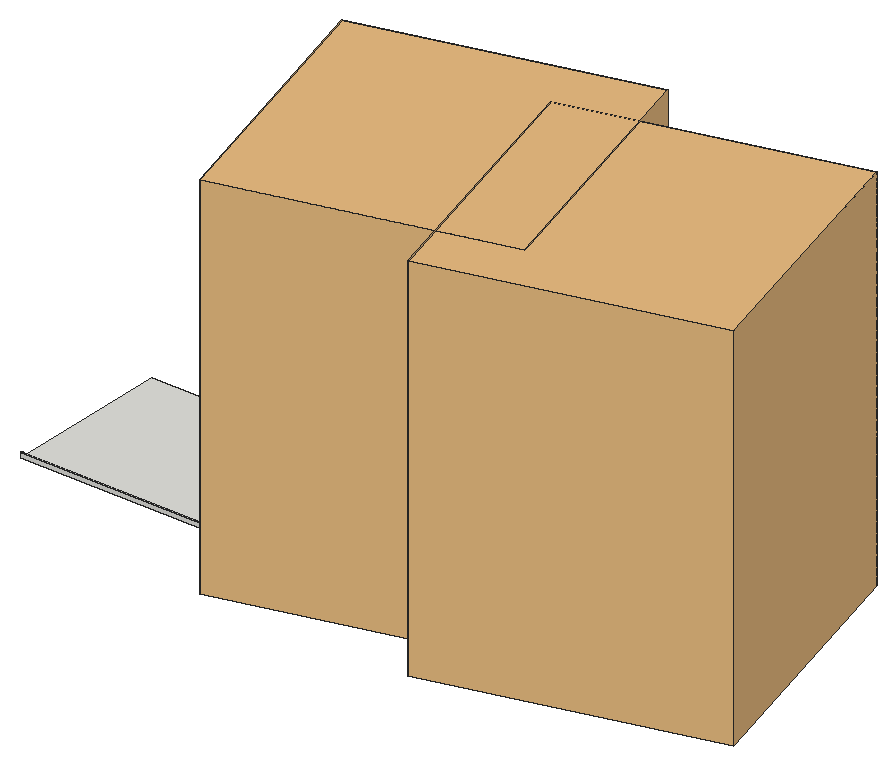
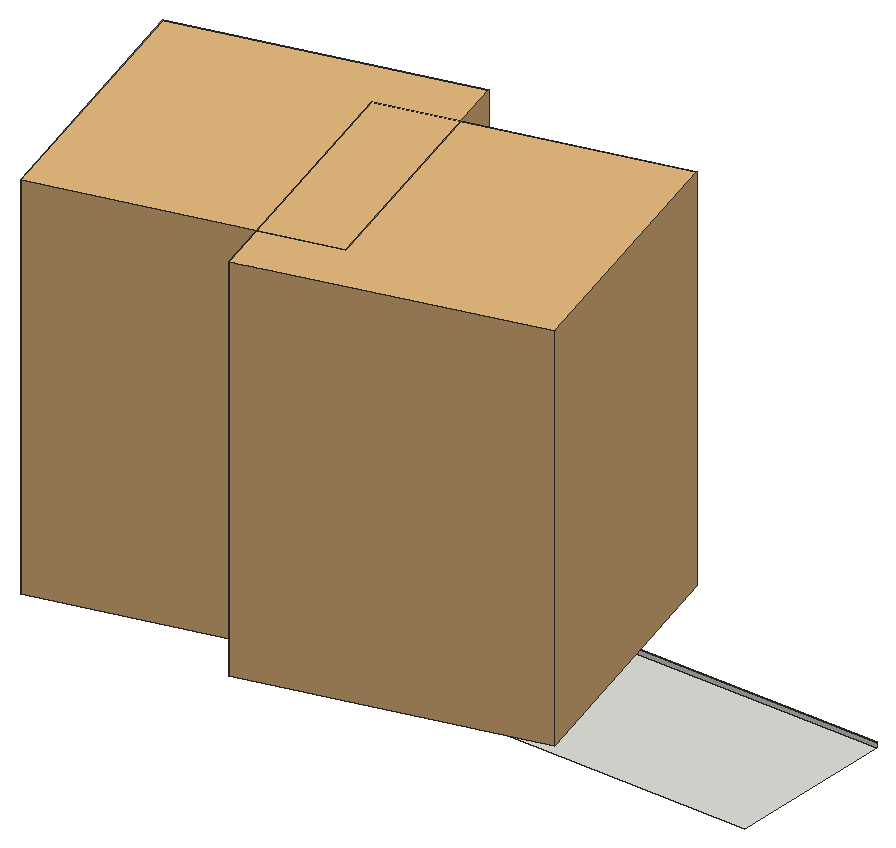
# SketchUp Ruby script. Lengths in inches.
U = 1.inch
M = Sketchup.active_model
def pt(a) = Geom::Point3d.new(a.map { |v| v * U })
def face(e, loops, mat)
  f = e.add_face(loops[0].map { |a| pt(a) })
  loops[1..].each { |l| e.add_face(l.map { |a| pt(a) }).erase! }
  f.material = f.back_material = mat if mat
  f
end
# faces: each face lists its corners as indices into pts; further lists are holes
def faces(e, pts, list, mat = nil) = list.each { |f| face(e, (f[0].is_a?(Array) ? f : [f]).map { |l| l.map { |i| pts[i] } }, mat) }
# xy, xz, yz: faces in a plane at the given z, y or x. An outline is a flat list of corners, or four numbers for a rectangle; further outlines are holes
def ring(l) = l.size == 4 ? [[l[0], l[1]], [l[2], l[1]], [l[2], l[3]], [l[0], l[3]]] : l.each_slice(2).to_a
def flat(e, list, mat, &to3) = list.each { |f| face(e, (f[0].is_a?(Array) ? f : [f]).map { |l| ring(l).map { |u, v| to3.(u, v) } }, mat) }
def xy(e, z, list, mat = nil) = flat(e, list, mat) { |x, y| [x, y, z] }
def xz(e, y, list, mat = nil) = flat(e, list, mat) { |x, z| [x, y, z] }
def yz(e, x, list, mat = nil) = flat(e, list, mat) { |y, z| [x, y, z] }
def lines(e, pts, list) = list.each { |a, b| e.add_line(pt(pts[a]), pt(pts[b])) }
# prism: a flat outline (further loops are holes) pulled along v
def prism(e, loops, v, mat = nil)
  f = face(e, loops, mat); d = Geom::Vector3d.new(v.map { |x| x * U })
  f.pushpull(f.normal.samedirection?(d) ? d.length : -d.length)
end
def box(e, o, s, mat = nil) = prism(e, [[o, [o[0] + s[0], o[1], o[2]], [o[0] + s[0], o[1] + s[1], o[2]], [o[0], o[1] + s[1], o[2]]]], [0, 0, s[2]], mat)
def at(x, y, z, deg = 0) = Geom::Transformation.translation(pt([x, y, z])) * Geom::Transformation.rotation(ORIGIN, Z_AXIS, deg.degrees)
def axes(o, x, y, z) = Geom::Transformation.new([*x, 0, *y, 0, *z, 0, *pt(o).to_a, 1])
def part(name) = M.definitions.add(name)
# library, detail: a bought-in or finely detailed component or shape, given as its bounding box
def library(name, o, s) = part(name).tap { |d| box(d.entities, o, s) }
def detail(e, o, s) = box(e.add_group.entities, o, s)
def put(e, d, t, mat = nil) = e.add_instance(d, t).tap { |i| i.material = mat if mat }
def group(e, t, mat = nil) = e.add_group.tap { |g| g.transformation = t; g.material = mat if mat }.entities
root = M.entities
M.materials.add("Material82").color = [68, 110, 58]
M.materials.add("Material83").color = [48, 90, 38]
M.materials.add("Material84").color = [68, 110, 48]
M.materials.add("Material85").color = [48, 90, 48]
M.materials.add("Material86").color = [58, 110, 58]
M.materials.add("Material87").color = [58, 90, 38]
M.materials.add("Material88").color = [68, 100, 58]
M.materials.add("Material89").color = [48, 100, 38]
c1 = part("grass00")
p = [[-0.6875,0.15,0],[-0.56,0.08,5.52],[-0.04,0.03,2.76],[0.48,-0.02,0],[0.35,-0.02,5.52],[-0.1,-0.14,5.52],
  [-0.12,0.65,8.37],[-0.42,0.65,8.37]]
faces(c1.entities,p,[[0,1,2,3],[3,2,4],[1,5,2],[5,4,2],[1,6,5],[4,5,6],[7,6,1]])
c2 = part("Group16\#1")
put(c2.entities,c1,axes([1.44,-0.61,-0.01],[0.05352,0.12609,0],[-0.10704,0.04543,0.07239],[0.06664,-0.02828,0.11628]),"Material85")
put(c2.entities,c1,axes([0.76,-0.15,-0.01],[0.04676,0.24062,0],[-0.23162,0.04501,0.06642],[0.0652,-0.01267,0.23595]),"Material82")
put(c2.entities,c1,axes([0.79,0.01,-0.01],[-0.00606,0.34651,0],[-0.34381,-0.00602,0.0432],[0.04319,0.00076,0.34386]))
put(c2.entities,c1,axes([1,0.23,-0.01],[-0.07192,0.31144,0],[-0.28722,-0.06632,0.1236],[0.12043,0.02781,0.29478]),"Material84")
put(c2.entities,c1,axes([1.66,0.77,-0.01],[-0.13828,0.29651,0],[-0.21551,-0.1005,0.22471],[0.20365,0.09498,0.23779]),"Material89")
put(c2.entities,c1,axes([0.6875,0.52,-0.01],[-0.18126,0.24051,0],[-0.22746,-0.17142,0.09788],[0.07817,0.05891,0.28481]),"Material84")
put(c2.entities,c1,axes([0.68,0.78,-0.01],[-0.215,0.18688,0],[-0.12385,-0.14248,0.21334],[0.13995,0.16101,0.18878]),"Material82")
put(c2.entities,c1,axes([0.56,1,-0.01],[-0.13756,0.07624,0],[-0.06159,-0.11112,0.0927],[0.04494,0.08108,0.12705]),"Material84")
put(c2.entities,c1,axes([0.2,0.64,-0.01],[-0.23729,0.07254,0],[-0.05711,-0.18681,0.153],[0.04473,0.14632,0.19535]),"Material89")
put(c2.entities,c1,axes([0.0625,0.72,-0.01],[-0.28874,0.02525,0],[-0.02179,-0.24916,0.14647],[0.01276,0.14591,0.25012]),"Material82")
put(c2.entities,c1,axes([-0.08,0.62,-0.01],[-0.34089,-0.04187,0],[0.03255,-0.26504,0.216],[-0.02633,0.21439,0.26703]),"Material89")
put(c2.entities,c1,axes([-0.34,0.98,-0.01],[-0.14314,-0.0493,0],[0.04397,-0.12769,0.06843],[-0.02228,0.0647,0.13505]),"Material89")
put(c2.entities,c1,axes([-0.87,1.45,-0.01],[-0.23488,-0.14114,0],[0.13761,-0.22901,0.06087],[-0.03135,0.05217,0.26717]))
put(c2.entities,c1,axes([-0.72,0.77,-0.01],[-0.14208,-0.13251,0],[0.07209,-0.0773,0.16301],[-0.11118,0.11922,0.1057]),"Material89")
put(c2.entities,c1,axes([-0.62,0.43,-0.01],[-0.14845,-0.21203,0],[0.18654,-0.13061,0.12304],[-0.10079,0.07057,0.22772]),"Material82")
put(c2.entities,c1,axes([-0.68,0.29,-0.01],[-0.13639,-0.32136,0],[0.31723,-0.13464,0.05579],[-0.05136,0.0218,0.34462]),"Material83")
put(c2.entities,c1,axes([-0.64,0.125,-0.01],[-0.0458,-0.23569,0],[0.22124,-0.043,0.08276],[-0.08124,0.01579,0.22538]),"Material86")
put(c2.entities,c1,axes([-1.6,-0.03,-0.01],[0.00576,-0.32897,0],[0.27526,0.00482,0.18018],[-0.18015,-0.00315,0.2753]),"Material84")
put(c2.entities,c1,axes([-1.36,-0.31,-0.01],[0.05718,-0.24765,0],[0.18172,0.04196,0.17267],[-0.16825,-0.03885,0.1865]),"Material89")
put(c2.entities,c1,axes([-1.54,-0.72,-0.01],[0.06537,-0.14017,0],[0.13555,0.06321,0.03939],[-0.0357,-0.01665,0.14956]))
put(c2.entities,c1,axes([-1.19,-0.9,-0.01],[0.09597,-0.12735,0],[0.11214,0.08451,0.07557],[-0.06035,-0.04548,0.14042]),"Material88")
put(c2.entities,c1,axes([-0.47,-0.54,-0.01],[0.11588,-0.10072,0],[0.0618,0.0711,0.12124],[-0.07953,-0.0915,0.0942]))
put(c2.entities,c1,axes([-0.47,-0.84,-0.01],[0.11927,-0.0661,0],[0.06603,0.11913,0.00646],[-0.00313,-0.00565,0.13621]),"Material84")
put(c2.entities,c1,axes([-0.38,-1.24,-0.01],[0.28037,-0.08571,0],[0.0618,0.20215,0.20315],[-0.05939,-0.19428,0.21139]),"Material88")
put(c2.entities,c1,axes([-0.06,-0.66,-0.01],[0.22719,-0.01987,0],[0.01247,0.14255,0.17758],[-0.01547,-0.17691,0.1431]),"Material87")
put(c2.entities,c1,axes([0.11,-0.89,-0.01],[0.14882,0.01828,0],[-0.01058,0.08611,0.12229],[0.01491,-0.12138,0.08676]),"Material85")
put(c2.entities,c1,axes([0.25,-0.72,-0.01],[0.20481,0.07053,0],[-0.06206,0.18022,0.10291],[0.03351,-0.0973,0.1906]),"Material85")
put(c2.entities,c1,axes([0.85,-1.42,-0.01],[0.16481,0.09904,0],[-0.09472,0.15762,0.05616],[0.02893,-0.04814,0.18389]),"Material84")
put(c2.entities,c1,axes([1.01,-1.09,-0.01],[0.21858,0.20385,0],[-0.17495,0.1876,0.15339],[0.10462,-0.11218,0.25652]),"Material89")
put(c2.entities,c1,axes([1.01,-0.71,-0.01],[0.08733,0.12473,0],[-0.06445,0.04512,0.13037],[0.1068,-0.07477,0.07867]),"Material85")
c3 = part("Group15\#1")
put(c3.entities,c2,at(0,0,0))
c4 = part("3darcstudiotree_grass00\#1")
put(c4.entities,c3,at(0,0,0))
c5 = library("Palm tree",[-4.09,-4.52,0],[193.52,193.51,258.93])
c6 = part("Palm+Tree")
put(c6.entities,c5,at(25.51,-21.81,0,15))
c7 = library("Group\#612",[0,0,0],[32.91,53.52,103.45])
xy(root,-42.1875,[[626.68,273.41,1048.66,387.84]])
xz(root,273.41,[[626.68,-42.1875,1048.66,-42.1875,1048.66,-38.61,848.97,-38.61,848.97,-39.125,626.68,-39.125],[626.68,-38.61,1048.66,-38.1875]])
put(root,c4,axes([808.61,334.13,-34.17],[-3.94658,0.83198,0],[-2.08533,-1.53849,-0.02635],[-0.05206,-0.03841,1.3895]))
put(root,c4,axes([807.23,326.65,-34.17],[2.20824,1.44568,0],[-4.06639,0.96604,-0.01693],[-0.06521,0.01549,1.59984]))
put(root,c4,axes([807.96,310.95,-34.17],[4.53975,0.53985,0],[-1.08694,1.4216,-0.04516],[-0.08333,0.10898,1.80387]))
put(root,c4,axes([808.67,323.88,-34.17],[-2.27595,1.46975,0],[-3.85308,-0.92798,-0.0342],[-0.14118,-0.034,1.63693]))
put(root,c4,axes([808.34,307.49,-34.17],[3.38368,1.04745,0],[-2.27938,1.14521,-0.02005],[-0.08327,0.04184,1.86077]))
put(root,c4,axes([810.4,335.1875,-34.17],[0.01113,-1.45353,0],[4.54919,0.00542,-0.03692],[0.17089,0.0002,1.57831]))
put(root,c4,axes([810.73,313.29,-34.17],[-1.2969,-1.20265,0],[3.80092,-0.63749,-0.01791],[0.10113,-0.01696,1.89984]))
put(root,c4,axes([810.83,291.65,-34.17],[0.25593,-1.38573,0],[3.33259,0.09573,-0.00937],[0.07232,0.00208,1.93766]))
put(root,c4,axes([810.72,287.07,-34.17],[-3.13946,0.49629,0],[-1.50487,-1.48058,-0.04281],[-0.09532,-0.09378,1.81418]))
put(root,c4,axes([810.62,329.8125,-34.17],[3.11316,-1.08854,0],[2.76667,1.23063,-0.03392],[0.0954,0.04244,1.32537]))
put(root,c4,axes([811.72,298.21,-34.17],[-3.90762,0.14516,0],[-0.37668,-1.57704,-0.0202],[-0.01231,-0.05153,1.95637]))
put(root,c4,axes([811.86,339.86,-34.17],[-1.14276,-1.73672,0],[3.49011,-0.35717,-0.03225],[0.18285,-0.01871,1.58326]))
put(root,c4,axes([810.58,282.42,-34.17],[3.63772,-0.04618,0],[0.1059,1.29755,-0.04101],[0.00733,0.08987,1.37186]))
put(root,c4,axes([810.64,337.85,-34.17],[0.13497,1.53866,0],[-3.75353,0.05121,-0.02489],[-0.17047,0.00233,1.9295]))
put(root,c4,axes([811.2,333.37,-34.17],[-2.50392,0.92561,0],[-3.00944,-1.26617,-0.02311],[-0.06646,-0.02796,1.38694]))
put(root,c4,axes([812.36,326.64,-34.17],[-4.13167,0.24366,0],[-0.69238,-1.82599,-0.06496],[-0.05165,-0.1362,1.88637]))
put(root,c4,axes([811.55,309.54,-34.17],[-1.70819,1.11812,0],[-3.96876,-0.943,-0.04504],[-0.21667,-0.05148,1.9506]))
put(root,c4,axes([811.74,318.65,-34.17],[3.79912,-1.05543,0],[2.19489,1.22878,-0.03692],[0.13668,0.07652,1.83631]))
put(root,c4,axes([811.61,284.9,-34.17],[3.28657,0.21022,0],[-0.53923,1.31117,-0.01255],[-0.01302,0.03166,1.63564]))
put(root,c4,axes([812.21,324.84,-34.17],[-2.37455,1.29783,0],[-2.73236,-0.77752,-0.00844],[-0.03827,-0.01089,1.41311]))
put(root,c4,axes([811.54,315.9,-34.17],[2.3712,1.21069,0],[-3.58151,1.09097,-0.04605],[-0.15475,0.04714,1.44046]))
put(root,c4,axes([812.77,301.02,-34.17],[1.66455,-1.14728,0],[3.31311,0.74761,-0.04415],[0.26641,0.06012,1.98924]))
put(root,c4,axes([813.87,331.24,-34.17],[-0.63027,-1.58552,0],[4.65732,-0.28794,-0.06318],[0.24644,-0.01524,1.39517]))
put(root,c4,axes([812.33,302.46,-34.17],[2.52471,1.58546,0],[-3.52346,0.87265,-0.052],[-0.25077,0.06211,1.7759]))
put(root,c4,axes([813.1,323.25,-34.17],[3.33412,-1.28398,0],[2.96352,1.19685,-0.04175],[0.14903,0.06019,1.62422]))
put(root,c4,axes([812.5,319.77,-34.17],[3.98735,0.11869,0],[-0.3473,1.81468,-0.00004],[-0.00002,0.00009,1.93334]))
put(root,c4,axes([814.15,294.22,-34.17],[-2.08457,-1.53905,0],[3.84719,-0.81044,-0.05822],[0.30315,-0.06386,1.92982]))
put(root,c4,axes([813.28,311.12,-34.17],[0.24653,1.78059,0],[-4.18646,0.09015,-0.05861],[-0.36644,0.00789,1.96776]))
put(root,c4,axes([812.78,305.77,-34.17],[4.09909,0.70116,0],[-1.55013,1.40946,-0.01845],[-0.03388,0.03081,1.34771]))
put(root,c4,axes([812.82,281.39,-34.17],[1.95248,1.61036,0],[-3.842,0.72449,-0.01048],[-0.04175,0.00787,1.40926]))
put(root,c4,axes([813.14,296.15,-34.17],[3.93599,0.37319,0],[-1.10472,1.81211,-0.03506],[-0.03066,0.05029,1.32515]))
put(root,c4,axes([813.79,289.81,-34.17],[3.76504,-0.34797,0],[1.07827,1.81452,-0.02268],[0.0226,0.03802,1.5468]))
put(root,c4,axes([813.79,306.82,-34.17],[-0.03028,1.81071,0],[-4.52004,-0.01176,-0.01347],[-0.05788,-0.00015,1.45625]))
put(root,c4,axes([816,288.28,-34.17],[2.88127,-0.83898,0],[2.47269,1.32072,-0.02283],[0.06307,0.03369,1.4512]))
put(root,c4,axes([816.92,293.27,-34.17],[-1.69688,-1.72936,0],[4.23511,-0.64631,-0.05475],[0.2829,-0.04317,1.88574]))
put(root,c4,axes([816,285.39,-34.17],[3.22121,-0.88629,0],[2.07064,1.17047,-0.00731],[0.02777,0.0157,1.80073]))
put(root,c4,axes([817.13,335.42,-34.17],[-1.90792,-1.42621,0],[3.47826,-0.72369,-0.03938],[0.16408,-0.03414,1.38871]))
put(root,c4,axes([816.19,322.01,-34.17],[3.56261,-0.94567,0],[1.87037,1.0959,-0.0013],[0.00431,0.00253,1.49257]))
put(root,c4,axes([816.1,296.77,-34.17],[-1.05565,1.36177,0],[-3.91341,-0.47183,-0.0271],[-0.14616,-0.01762,1.72974]))
put(root,c4,axes([817.39,289.4375,-34.17],[-4.0685,0.50795,0],[-1.17773,-1.46714,-0.03323],[-0.06082,-0.07576,1.77353]))
put(root,c4,axes([816.45,282.8,-34.17],[4.25936,0.17724,0],[-0.36955,1.38123,-0.03171],[-0.02162,0.08082,1.71518]))
put(root,c4,axes([818.06,299.0625,-34.17],[0.20903,-1.7077,0],[3.89534,0.07416,-0.00402],[0.01821,0.00035,1.3243]))
put(root,c4,axes([818.17,305.18,-34.17],[-3.49989,-0.62042,0],[1.34924,-1.18377,-0.02079],[0.0557,-0.04887,1.61237]))
put(root,c4,axes([817.42,307.34,-34.17],[-2.24971,1.27376,0],[-2.901,-0.79689,-0.01437],[-0.08541,-0.02346,1.91898]))
put(root,c4,axes([818.32,329.74,-34.17],[-2.13915,-1.27276,0],[3.26215,-0.85272,-0.05028],[0.27845,-0.07279,1.94898]))
put(root,c4,axes([817.19,333.7,-34.17],[4.02195,-0.32221,0],[0.68718,1.33408,-0.00331],[0.00405,0.00786,1.58887]))
put(root,c4,axes([816.6875,320,-34.17],[4.32701,0.55712,0],[-1.36775,1.65217,-0.00124],[-0.00192,0.00232,1.65228]))
put(root,c4,axes([817.89,327.39,-34.17],[-1.63539,1.16071,0],[-3.40916,-0.74706,-0.05151],[-0.29339,-0.06429,1.90487]))
put(root,c4,axes([817.09,324.48,-34.17],[1.01762,1.37596,0],[-4.26505,0.49058,-0.00405],[-0.01582,0.00182,1.35389]))
put(root,c4,axes([819.38,316.36,-34.17],[-3.3697,-1.02042,0],[2.44227,-1.25434,-0.00705],[0.02625,-0.01348,1.8369]))
put(root,c4,axes([818.52,317.9375,-34.17],[2.02024,-1.18426,0],[3.76291,0.99837,-0.06298],[0.20491,0.05437,1.33293]))
put(root,c4,axes([817.74,281.31,-34.17],[4.3094,-0.16311,0],[0.42718,1.75528,-0.01064],[0.00539,0.02213,1.77558]))
put(root,c4,axes([819.51,331.57,-34.17],[-2.95002,-1.42448,0],[3.56758,-1.14909,-0.03335],[0.13906,-0.04479,1.85855]))
put(root,c4,axes([818.93,312.33,-34.17],[0.35372,-1.85816,0],[4.64402,0.13749,-0.06273],[0.35272,0.01044,1.9684]))
put(root,c4,axes([818.52,291.29,-34.17],[-1.74852,1.13217,0],[-3.21789,-0.77293,-0.03041],[-0.12145,-0.02917,1.3205]))
put(root,c4,axes([819.84,310.09,-34.17],[-1.80602,-1.23313,0],[3.1704,-0.72217,-0.00817],[0.04009,-0.00913,1.55447]))
put(root,c4,axes([818.12,338.45,-34.17],[3.63959,0.40285,0],[-0.8944,1.25675,-0.00495],[-0.00749,0.01053,1.38942]))
put(root,c4,axes([819.09,313.01,-34.17],[3.72507,-0.62439,0],[1.73357,1.60854,-0.00549],[0.00931,0.00864,1.44062]))
put(root,c4,axes([819.08,301.21,-34.17],[3.99736,-0.43263,0],[1.22188,1.75587,-0.05143],[0.05673,0.08152,1.44218]))
put(root,c4,axes([819.05,303.03,-34.17],[-0.70731,1.48216,0],[-4.42453,-0.32839,-0.01956],[-0.1033,-0.00767,1.8138]))
put(root,c4,axes([821.52,298.91,-34.17],[-4.33089,0.41445,0],[-1.11243,-1.80796,-0.06662],[-0.06204,-0.10083,1.39642]))
put(root,c4,axes([822.41,289.05,-34.17],[-3.26976,-0.5137,0],[1.67175,-1.65498,-0.00121],[0.00254,-0.00252,1.92636]))
put(root,c4,axes([821.64,333.375,-34.17],[1.4091,-1.17417,0],[3.00858,0.56155,-0.04441],[0.31581,0.05895,1.96303]))
put(root,c4,axes([822.39,329.09,-34.17],[-0.33318,-1.39627,0],[3.47077,-0.12881,-0.04952],[0.2452,-0.0091,1.29958]))
put(root,c4,axes([822.5,324.74,-34.17],[-3.53744,1.16554,0],[-2.5606,-1.20869,-0.03098],[-0.10582,-0.04995,1.59479]))
put(root,c4,axes([823.11,337.18,-34.17],[-3.84526,-0.22431,0],[0.50015,-1.33348,-0.00812],[0.00644,-0.01718,1.3892]))
put(root,c4,axes([822.63,319.86,-34.17],[-3.00421,0.76942,0],[-2.15411,-1.30812,-0.04277],[-0.14646,-0.08894,1.86401]))
put(root,c4,axes([822.09,291.51,-34.17],[-0.58592,1.57945,0],[-3.44253,-0.19862,-0.02144],[-0.15876,-0.00916,1.9513]))
put(root,c4,axes([822.6,312.34,-34.17],[-3.04736,0.88871,0],[-2.40783,-1.28411,-0.01371],[-0.03527,-0.01881,1.31321]))
put(root,c4,axes([822.09,331.78,-34.17],[3.34176,-0.01383,0],[0.04057,1.52455,-0.01029],[0.00052,0.01945,1.389]))
put(root,c4,axes([823.22,296.11,-34.17],[1.49416,-1.17809,0],[3.55261,0.70077,-0.01805],[0.08589,0.01694,1.58457]))
put(root,c4,axes([822.34,318.32,-34.17],[3.91979,-0.74164,0],[1.60866,1.32236,-0.04597],[0.11253,0.0925,1.57738]))
put(root,c4,axes([822.52,315.58,-34.17],[-2.1963,1.32957,0],[-3.96988,-1.01993,-0.00953],[-0.0332,-0.00853,1.47621]))
put(root,c4,axes([823.78,335.79,-34.17],[0.96851,-1.36822,0],[3.89034,0.4283,-0.00232],[0.01298,0.00143,1.76107]))
put(root,c4,axes([822.77,322.77,-34.17],[3.27047,-0.2692,0],[0.72961,1.37861,-0.04941],[0.05481,0.10356,1.4533]))
put(root,c4,axes([824,305.79,-34.17],[2.10515,-1.21949,0],[3.30844,0.88826,-0.01892],[0.09087,0.0244,1.74337]))
put(root,c4,axes([823.88,284.625,-34.17],[-2.16702,1.28274,0],[-3.03597,-0.79769,-0.03773],[-0.16249,-0.04269,1.41517]))
put(root,c4,axes([823.11,326.65,-34.17],[4.03817,0.43694,0],[-1.08149,1.5545,-0.02738],[-0.04454,0.06402,1.88342]))
put(root,c4,axes([823.66,312.99,-34.17],[4.33985,-0.71517,0],[1.81915,1.7169,-0.05614],[0.0962,0.09079,1.57175]))
put(root,c4,axes([824.68,301.33,-34.17],[1.94166,-1.68054,0],[3.68889,0.66287,-0.02827],[0.1643,0.02952,1.94019]))
put(root,c4,axes([823.99,307.22,-34.17],[0.75441,1.71197,0],[-3.26624,0.22386,-0.03272],[-0.2394,0.01641,1.8454]))
put(root,c4,axes([823.72,309.46,-34.17],[2.94946,0.97112,0],[-2.79078,1.31828,-0.05497],[-0.191,0.09022,1.76958]))
put(root,c4,axes([823.69,302.05,-34.17],[2.19107,1.06462,0],[-2.74426,0.87841,-0.00448],[-0.02021,0.00647,1.5389]))
put(root,c4,axes([824.85,294.37,-34.17],[2.33071,-1.20912,0],[3.74929,1.12403,-0.05929],[0.20074,0.06018,1.50135]))
put(root,c4,axes([824.59,283.1,-34.17],[-0.50717,1.45325,0],[-4.1597,-0.22578,-0.0385],[-0.18859,-0.01024,1.55608]))
put(root,c4,axes([824.98,287.78,-34.17],[4.27397,-0.60338,0],[1.4489,1.5962,-0.05713],[0.08848,0.09748,1.48067]))
put(root,c4,axes([827.03,326.3,-34.17],[-2.9256,-1.47399,0],[3.63184,-1.12114,-0.01534],[0.06015,-0.01857,1.72134]))
put(root,c4,axes([826.8125,311.77,-34.17],[-4.1987,0.12334,0],[-0.25997,-1.37638,-0.0204],[-0.0079,-0.04182,1.3669]))
put(root,c4,axes([827.18,330.98,-34.17],[-4.00085,-0.57986,0],[1.27846,-1.37193,-0.00277],[0.00474,-0.00509,1.38049]))
put(root,c4,axes([827.71,314.24,-34.17],[-3.39001,-0.81782,0],[2.4179,-1.55881,-0.03935],[0.08518,-0.05492,1.44076]))
put(root,c4,axes([827.02,287.1,-34.17],[3.84648,-0.75898,0],[1.52103,1.1989,-0.01525],[0.0428,0.03373,1.59832]))
put(root,c4,axes([827.66,320.33,-34.17],[2.20697,-0.9726,0],[2.75858,0.97355,-0.01984],[0.09708,0.03426,1.82222]))
put(root,c4,axes([827.47,315.36,-34.17],[0.68368,1.71904,0],[-3.38759,0.20954,-0.03929],[-0.29518,0.01826,1.95437]))
put(root,c4,axes([828.95,322.4375,-34.17],[-2.04632,-1.05436,0],[3.10393,-0.93693,-0.02737],[0.09658,-0.02915,1.30175]))
put(root,c4,axes([827.87,308.98,-34.17],[-0.28903,1.73584,0],[-3.34699,-0.08668,-0.03425],[-0.21957,-0.00569,1.61497]))
put(root,c4,axes([828.71,329.46,-34.17],[1.71259,-1.30416,0],[3.53393,0.72176,-0.01075],[0.04765,0.00973,1.48923]))
put(root,c4,axes([828.99,295.62,-34.17],[-3.772,0.03773,0],[-0.10384,-1.61464,-0.00196],[-0.00024,-0.00377,1.49745]))
put(root,c4,axes([828.33,290.01,-34.17],[-2.36342,1.1502,0],[-3.36153,-1.07427,-0.04128],[-0.15124,-0.04833,1.52936]))
put(root,c4,axes([827.9,294.41,-34.17],[4.05183,0.05747,0],[-0.14664,1.60785,-0.02702],[-0.00634,0.06949,1.99535]))
put(root,c4,axes([828.81,338.34,-34.17],[2.29885,-0.96399,0],[2.83055,1.04983,-0.02136],[0.08662,0.03213,1.62144]))
put(root,c4,axes([829.53,292.19,-34.17],[-4.17405,-0.19289,0],[0.40333,-1.35747,-0.00847],[0.00693,-0.02334,1.82708]))
put(root,c4,axes([828.48,318.61,-34.17],[1.65421,1.20964,0],[-3.07102,0.65317,-0.03445],[-0.21317,0.04534,1.83855]))
put(root,c4,axes([830.18,286.15,-34.17],[-2.90823,-0.76432,0],[2.41266,-1.42777,-0.04785],[0.14851,-0.08788,1.82518]))
put(root,c4,axes([829.21,305.75,-34.17],[-1.04428,1.44728,0],[-3.25699,-0.36551,-0.00052],[-0.00331,-0.00037,1.67384]))
put(root,c4,axes([829.34,306.83,-34.17],[3.83018,0.17914,0],[-0.49889,1.65896,-0.05841],[-0.02825,0.09394,1.30397]))
put(root,c4,axes([830.86,299.99,-34.17],[-3.60335,-0.2844,0],[0.69529,-1.3701,-0.00178],[0.00231,-0.00455,1.75352]))
put(root,c4,axes([830.3125,324.37,-34.17],[-2.93874,0.89671,0],[-2.33959,-1.1925,-0.04163],[-0.12402,-0.06321,1.39503]))
put(root,c4,axes([829.45,333.02,-34.17],[2.61631,0.861,0],[-2.17217,1.02658,-0.00812],[-0.03307,0.01563,1.6158]))
put(root,c4,axes([829.41,298.75,-34.17],[2.19518,1.25426,0],[-3.21279,0.87453,-0.02215],[-0.10628,0.02893,1.70619]))
put(root,c4,axes([830.09,282.39,-34.17],[0.43339,1.54675,0],[-3.36238,0.14653,-0.03685],[-0.25104,0.01094,1.73767]))
put(root,c4,axes([830.26,339.96,-34.17],[3.63873,-0.8009,0],[1.86273,1.31624,-0.03495],[0.11311,0.07993,1.90256]))
put(root,c4,axes([829.71,334.85,-34.17],[3.82301,1.06562,0],[-2.5922,1.44638,-0.0169],[-0.04207,0.02347,1.45184]))
put(root,c4,axes([830.66,302.78,-34.17],[3.73956,-0.25134,0],[0.58802,1.36068,-0.03176],[0.03776,0.08738,1.85682]))
put(root,c4,axes([832.53,295.76,-34.17],[-2.3605,-1.50274,0],[2.8114,-0.68684,-0.00146],[0.00663,-0.00162,1.32424]))
put(root,c4,axes([832.49,290.26,-34.17],[3.76532,-0.82989,0],[2.11238,1.49062,-0.04605],[0.09606,0.06778,1.38783]))
put(root,c4,axes([833.75,287.23,-34.17],[-2.75712,-0.97177,0],[2.36987,-1.04575,-0.04195],[0.16334,-0.07208,1.55746]))
put(root,c4,axes([832.32,333.26,-34.17],[1.13904,1.65719,0],[-4.07352,0.43546,-0.03421],[-0.20227,0.02162,1.93796]))
put(root,c4,axes([834.32,303.49,-34.17],[-1.0442,-1.68413,0],[4.42012,-0.42624,-0.03172],[0.12352,-0.01191,1.36741]))
put(root,c4,axes([834.48,283.2,-34.17],[-2.93582,-0.70247,0],[2.08855,-1.35755,-0.00574],[0.01328,-0.00863,1.3472]))
put(root,c4,axes([834.5,312.27,-34.17],[-2.87675,-1.09055,0],[2.6601,-1.09136,-0.02949],[0.13969,-0.05731,1.96656]))
put(root,c4,axes([834.64,317.73,-34.17],[-2.96111,-1.38906,0],[2.74036,-0.90856,-0.02964],[0.13819,-0.04582,1.63454]))
put(root,c4,axes([833.05,301.13,-34.17],[2.75422,1.28702,0],[-2.68657,0.89417,-0.05003],[-0.26479,0.08813,1.82479]))
put(root,c4,axes([833.21,307.34,-34.17],[2.36808,1.36159,0],[-2.95794,0.80011,-0.03781],[-0.20263,0.05481,1.74723]))
put(root,c4,axes([833.27,335.56,-34.17],[4.47082,0.11069,0],[-0.26321,1.65346,-0.04601],[-0.01202,0.07548,1.31249]))
put(root,c4,axes([833.91,316.08,-34.17],[-2.49032,1.32428,0],[-3.19574,-0.93467,-0.0152],[-0.05407,-0.01581,1.3203]))
put(root,c4,axes([833.36,308.59,-34.17],[1.04539,1.48143,0],[-4.29845,0.47176,-0.02844],[-0.1492,0.01637,1.82107]))
put(root,c4,axes([834.14,329.1,-34.17],[-2.32252,1.56487,0],[-3.68383,-0.85034,-0.03733],[-0.14959,-0.03453,1.48568]))
put(root,c4,axes([833.53,323.96,-34.17],[2.07418,1.09295,0],[-3.13936,0.92662,-0.0157],[-0.06877,0.0203,1.60759]))
put(root,c4,axes([834.23,304.39,-34.17],[3.63146,-0.94763,0],[2.16895,1.29272,-0.03005],[0.10609,0.06323,1.88475]))
put(root,c4,axes([833.59,339.45,-34.17],[4.62364,0.41674,0],[-0.83657,1.44354,-0.00333],[-0.00361,0.00623,1.36941]))
put(root,c4,axes([833.82,314.51,-34.17],[0.90968,1.754,0],[-3.81846,0.30801,-0.01369],[-0.06439,0.00519,1.40267]))
put(root,c4,axes([834.41,285.43,-34.17],[0.278,1.64734,0],[-3.85699,0.10123,-0.01024],[-0.06423,0.00169,1.82096]))
put(root,c4,axes([834.91,321.67,-34.17],[-1.2304,1.69187,0],[-3.83777,-0.43408,-0.02925],[-0.12783,-0.01446,1.36051]))
put(root,c4,axes([834.58,327.29,-34.17],[2.50159,1.07866,0],[-2.96417,1.06917,-0.03451],[-0.16033,0.05783,1.89576]))
put(root,c4,axes([834.72,331.67,-34.17],[3.85299,0.72056,0],[-1.4234,1.18377,-0.0026],[-0.00811,0.00675,1.81639]))
put(root,c4,axes([836.28,294.17,-34.17],[-3.94572,0.20967,0],[-0.54102,-1.58348,-0.01091],[-0.00895,-0.02619,1.8656]))
put(root,c4,axes([834.92,291.15,-34.17],[4.67805,0.10708,0],[-0.2535,1.72242,-0.0212],[-0.00736,0.05004,1.96575]))
put(root,c4,axes([835.21,319.91,-34.17],[3.89819,0.51903,0],[-1.48599,1.73579,-0.0473],[-0.0826,0.09649,1.90097]))
put(root,c4,axes([835.27,338.21,-34.17],[3.72345,0.43237,0],[-1.05501,1.41306,-0.01058],[-0.0164,0.02196,1.53588]))
put(root,c4,axes([835.44,298.4,-34.17],[3.62609,0.38691,0],[-0.94095,1.37154,-0.04799],[-0.07441,0.10847,1.60328]))
put(root,c4,axes([838.53,287.81,-34.17],[-2.74827,-0.90606,0],[2.5057,-1.18207,-0.04185],[0.15974,-0.07536,1.7425]))
put(root,c4,axes([838.8125,319.83,-34.17],[-2.21298,-1.13198,0],[3.27865,-0.99688,-0.03514],[0.15829,-0.04813,1.76492]))
put(root,c4,axes([838.75,331.16,-34.17],[1.56077,-1.21628,0],[3.51485,0.70149,-0.00728],[0.02929,0.00585,1.33141]))
put(root,c4,axes([838.24,333.29,-34.17],[-1.38329,1.54062,0],[-3.20389,-0.44741,-0.04758],[-0.27737,-0.03873,1.57537]))
put(root,c4,axes([839.29,291.96,-34.17],[-4.11808,-0.53305,0],[1.24091,-1.491,-0.0393],[0.07027,-0.08443,1.71017]))
put(root,c4,axes([838.86,322.96,-34.17],[-3.99092,0.85507,0],[-1.6879,-1.22527,-0.00649],[-0.01661,-0.01206,1.42064]))
put(root,c4,axes([838.21,335.81,-34.17],[-0.13254,1.67215,0],[-3.60359,-0.04442,-0.04056],[-0.20717,-0.00255,1.38085]))
put(root,c4,axes([839.06,302.03,-34.17],[-1.8566,1.22673,0],[-3.23788,-0.76215,-0.0186],[-0.08298,-0.01953,1.46845]))
put(root,c4,axes([839.24,312.94,-34.17],[3.63516,-0.37062,0],[1.04175,1.58916,-0.04398],[0.06662,0.10163,1.88821]))
put(root,c4,axes([839.19,283.5,-34.17],[4.38242,0.53414,0],[-1.34963,1.72221,-0.04987],[-0.06942,0.08859,1.61513]))
put(root,c6,at(783.57,232.43,-34.17))
put(root,c7,axes([951.26,235.4,-34.17],[1.13014,0.75656,0],[-0.75656,1.13014,0],[0,0,1.36]))
put(root,c6,at(928.95,232.43,-34.17))
